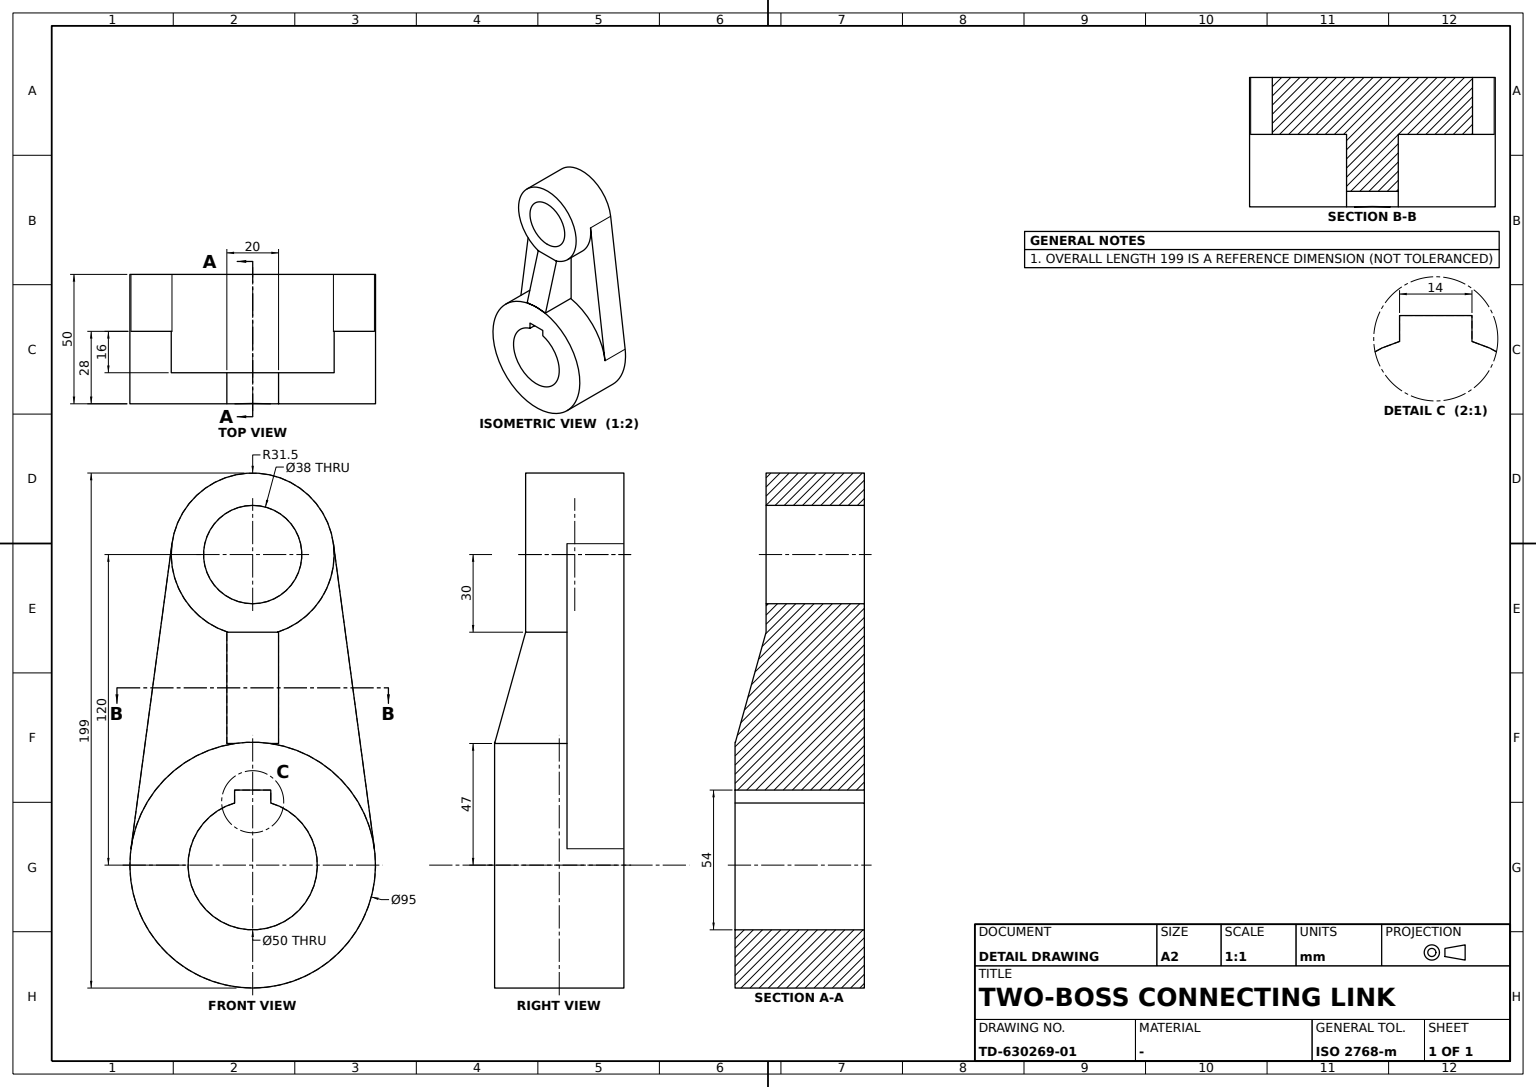
ISO-10303-21;
HEADER;
FILE_DESCRIPTION((''),'2;1');
FILE_NAME('','',(''),(''),'','','');
FILE_SCHEMA(('AUTOMOTIVE_DESIGN'));
ENDSEC;
DATA;
#1=APPLICATION_CONTEXT('');
#2=PRODUCT_CONTEXT('',#1,'mechanical');
#3=PRODUCT('','','',(#2));
#4=PRODUCT_DEFINITION_FORMATION('','',#3);
#5=PRODUCT_DEFINITION_CONTEXT('',#1,'design');
#6=PRODUCT_DEFINITION('','',#4,#5);
#7=PRODUCT_DEFINITION_SHAPE('','',#6);
#8=(LENGTH_UNIT()NAMED_UNIT(*)SI_UNIT(.MILLI.,.METRE.));
#9=(NAMED_UNIT(*)PLANE_ANGLE_UNIT()SI_UNIT($,.RADIAN.));
#10=(NAMED_UNIT(*)SI_UNIT($,.STERADIAN.)SOLID_ANGLE_UNIT());
#11=UNCERTAINTY_MEASURE_WITH_UNIT(LENGTH_MEASURE(0.005),#8,'distance_accuracy_value','');
#12=(GEOMETRIC_REPRESENTATION_CONTEXT(3)GLOBAL_UNCERTAINTY_ASSIGNED_CONTEXT((#11))GLOBAL_UNIT_ASSIGNED_CONTEXT((#8,#9,#10))REPRESENTATION_CONTEXT('',''));
#13=CARTESIAN_POINT('',(-25.,47.075884,6.333333));
#14=VERTEX_POINT('',#13);
#15=CARTESIAN_POINT('',(-3.,47.075884,6.333333));
#16=VERTEX_POINT('',#15);
#17=CARTESIAN_POINT('',(0.,47.075884,6.333333));
#18=DIRECTION('',(1.,0.,0.));
#19=VECTOR('',#18,1000.);
#20=LINE('',#17,#19);
#21=EDGE_CURVE('',#14,#16,#20,.T.);
#22=ORIENTED_EDGE('',*,*,#21,.F.);
#23=CARTESIAN_POINT('',(-25.,31.218744,124.2));
#24=VERTEX_POINT('',#23);
#25=DIRECTION('',(0.,-0.133333333,0.99107125));
#26=VECTOR('',#25,1000.);
#27=LINE('',#13,#26);
#28=EDGE_CURVE('',#14,#24,#27,.T.);
#29=ORIENTED_EDGE('',*,*,#28,.T.);
#30=CARTESIAN_POINT('',(-3.,31.218744,124.2));
#31=VERTEX_POINT('',#30);
#32=CARTESIAN_POINT('',(5.,31.218744,124.2));
#33=LINE('',#32,#19);
#34=EDGE_CURVE('',#24,#31,#33,.T.);
#35=ORIENTED_EDGE('',*,*,#34,.T.);
#36=LINE('',#15,#26);
#37=EDGE_CURVE('',#16,#31,#36,.T.);
#38=ORIENTED_EDGE('',*,*,#37,.F.);
#39=EDGE_LOOP('',(#22,#29,#35,#38));
#40=FACE_BOUND('',#39,.T.);
#41=DIRECTION('',(0.,0.99107125,0.133333333));
#42=AXIS2_PLACEMENT_3D('',#13,#41,#25);
#43=PLANE('',#42);
#44=ADVANCED_FACE('',(#40),#43,.T.);
#45=CARTESIAN_POINT('',(-25.,-31.218744,124.2));
#46=VERTEX_POINT('',#45);
#47=CARTESIAN_POINT('',(-3.,-31.218744,124.2));
#48=VERTEX_POINT('',#47);
#49=CARTESIAN_POINT('',(5.,-31.218744,124.2));
#50=LINE('',#49,#19);
#51=EDGE_CURVE('',#46,#48,#50,.T.);
#52=ORIENTED_EDGE('',*,*,#51,.T.);
#53=CARTESIAN_POINT('',(-3.,-9.604686,90.));
#54=VERTEX_POINT('',#53);
#55=CARTESIAN_POINT('',(-3.,0.,120.));
#56=DIRECTION('',(-1.,0.,0.));
#57=DIRECTION('',(0.,0.,1.));
#58=AXIS2_PLACEMENT_3D('',#55,#56,#57);
#59=CIRCLE('',#58,31.5);
#60=EDGE_CURVE('',#48,#54,#59,.F.);
#61=ORIENTED_EDGE('',*,*,#60,.T.);
#62=CARTESIAN_POINT('',(13.,-9.604686,90.));
#63=VERTEX_POINT('',#62);
#64=LINE('',#53,#19);
#65=EDGE_CURVE('',#63,#54,#64,.F.);
#66=ORIENTED_EDGE('',*,*,#65,.F.);
#67=CARTESIAN_POINT('',(13.,9.604686,90.));
#68=VERTEX_POINT('',#67);
#69=CARTESIAN_POINT('',(13.,0.,120.));
#70=DIRECTION('',(0.,0.,-1.));
#71=AXIS2_PLACEMENT_3D('',#69,#18,#70);
#72=CIRCLE('',#71,31.5);
#73=EDGE_CURVE('',#68,#63,#72,.T.);
#74=ORIENTED_EDGE('',*,*,#73,.F.);
#75=CARTESIAN_POINT('',(-3.,9.604686,90.));
#76=VERTEX_POINT('',#75);
#77=LINE('',#75,#19);
#78=EDGE_CURVE('',#76,#68,#77,.T.);
#79=ORIENTED_EDGE('',*,*,#78,.F.);
#80=EDGE_CURVE('',#76,#31,#59,.F.);
#81=ORIENTED_EDGE('',*,*,#80,.T.);
#82=ORIENTED_EDGE('',*,*,#34,.F.);
#83=CARTESIAN_POINT('',(-25.,0.,120.));
#84=AXIS2_PLACEMENT_3D('',#83,#18,#70);
#85=CIRCLE('',#84,31.5);
#86=EDGE_CURVE('',#46,#24,#85,.F.);
#87=ORIENTED_EDGE('',*,*,#86,.F.);
#88=EDGE_LOOP('',(#52,#61,#66,#74,#79,#81,#82,#87));
#89=FACE_BOUND('',#88,.T.);
#90=CARTESIAN_POINT('',(5.,0.,120.));
#91=DIRECTION('',(0.,1.,0.));
#92=AXIS2_PLACEMENT_3D('',#90,#18,#91);
#93=CYLINDRICAL_SURFACE('',#92,31.5);
#94=ADVANCED_FACE('',(#89),#93,.T.);
#95=CARTESIAN_POINT('',(25.,-10.,47.));
#96=VERTEX_POINT('',#95);
#97=CARTESIAN_POINT('',(-3.,-10.,47.));
#98=VERTEX_POINT('',#97);
#99=CARTESIAN_POINT('',(0.,-10.,47.));
#100=VECTOR('',#56,1000.);
#101=LINE('',#99,#100);
#102=EDGE_CURVE('',#96,#98,#101,.T.);
#103=ORIENTED_EDGE('',*,*,#102,.F.);
#104=CARTESIAN_POINT('',(13.,-10.,90.));
#105=VERTEX_POINT('',#104);
#106=CARTESIAN_POINT('',(35.362268,-10.,9.86854));
#107=DIRECTION('',(0.268798968,0.,-0.963196301));
#108=VECTOR('',#107,1000.);
#109=LINE('',#106,#108);
#110=EDGE_CURVE('',#105,#96,#109,.T.);
#111=ORIENTED_EDGE('',*,*,#110,.F.);
#112=CARTESIAN_POINT('',(-3.,-10.,90.));
#113=VERTEX_POINT('',#112);
#114=CARTESIAN_POINT('',(0.,-10.,90.));
#115=LINE('',#114,#19);
#116=EDGE_CURVE('',#113,#105,#115,.T.);
#117=ORIENTED_EDGE('',*,*,#116,.F.);
#118=CARTESIAN_POINT('',(-3.,-10.,0.));
#119=VECTOR('',#57,1000.);
#120=LINE('',#118,#119);
#121=EDGE_CURVE('',#98,#113,#120,.T.);
#122=ORIENTED_EDGE('',*,*,#121,.F.);
#123=EDGE_LOOP('',(#103,#111,#117,#122));
#124=FACE_BOUND('',#123,.T.);
#125=CARTESIAN_POINT('',(0.,-10.,0.));
#126=AXIS2_PLACEMENT_3D('',#125,#91,#56);
#127=PLANE('',#126);
#128=ADVANCED_FACE('',(#124),#127,.F.);
#129=CARTESIAN_POINT('',(-25.,0.,101.));
#130=VERTEX_POINT('',#129);
#131=CIRCLE('',#84,19.);
#132=EDGE_CURVE('',#130,#130,#131,.T.);
#133=ORIENTED_EDGE('',*,*,#132,.T.);
#134=EDGE_LOOP('',(#133));
#135=FACE_BOUND('',#134,.T.);
#136=CARTESIAN_POINT('',(-25.,7.,29.));
#137=VERTEX_POINT('',#136);
#138=CARTESIAN_POINT('',(-25.,7.,24.));
#139=VERTEX_POINT('',#138);
#140=CARTESIAN_POINT('',(-25.,7.,0.));
#141=VECTOR('',#70,1000.);
#142=LINE('',#140,#141);
#143=EDGE_CURVE('',#137,#139,#142,.T.);
#144=ORIENTED_EDGE('',*,*,#143,.F.);
#145=CARTESIAN_POINT('',(-25.,-7.,29.));
#146=VERTEX_POINT('',#145);
#147=CARTESIAN_POINT('',(-25.,0.,29.));
#148=VECTOR('',#91,1000.);
#149=LINE('',#147,#148);
#150=EDGE_CURVE('',#146,#137,#149,.T.);
#151=ORIENTED_EDGE('',*,*,#150,.F.);
#152=CARTESIAN_POINT('',(-25.,-7.,24.));
#153=VERTEX_POINT('',#152);
#154=CARTESIAN_POINT('',(-25.,-7.,0.));
#155=LINE('',#154,#119);
#156=EDGE_CURVE('',#153,#146,#155,.T.);
#157=ORIENTED_EDGE('',*,*,#156,.F.);
#158=CARTESIAN_POINT('',(-25.,0.,0.));
#159=AXIS2_PLACEMENT_3D('',#158,#18,#70);
#160=CIRCLE('',#159,25.);
#161=EDGE_CURVE('',#153,#139,#160,.T.);
#162=ORIENTED_EDGE('',*,*,#161,.T.);
#163=EDGE_LOOP('',(#144,#151,#157,#162));
#164=FACE_BOUND('',#163,.T.);
#165=ORIENTED_EDGE('',*,*,#28,.F.);
#166=CARTESIAN_POINT('',(-25.,-47.075884,6.333333));
#167=VERTEX_POINT('',#166);
#168=CIRCLE('',#159,47.5);
#169=EDGE_CURVE('',#167,#14,#168,.T.);
#170=ORIENTED_EDGE('',*,*,#169,.F.);
#171=DIRECTION('',(0.,-0.133333333,-0.99107125));
#172=VECTOR('',#171,1000.);
#173=LINE('',#166,#172);
#174=EDGE_CURVE('',#46,#167,#173,.T.);
#175=ORIENTED_EDGE('',*,*,#174,.F.);
#176=ORIENTED_EDGE('',*,*,#86,.T.);
#177=EDGE_LOOP('',(#165,#170,#175,#176));
#178=FACE_BOUND('',#177,.T.);
#179=AXIS2_PLACEMENT_3D('',#158,#18,#91);
#180=PLANE('',#179);
#181=ADVANCED_FACE('',(#135,#164,#178),#180,.F.);
#182=CARTESIAN_POINT('',(13.,10.,90.));
#183=VERTEX_POINT('',#182);
#184=CARTESIAN_POINT('',(13.,0.,90.));
#185=LINE('',#184,#148);
#186=EDGE_CURVE('',#68,#183,#185,.T.);
#187=ORIENTED_EDGE('',*,*,#186,.T.);
#188=CARTESIAN_POINT('',(-3.,10.,90.));
#189=VERTEX_POINT('',#188);
#190=CARTESIAN_POINT('',(0.,10.,90.));
#191=LINE('',#190,#19);
#192=EDGE_CURVE('',#189,#183,#191,.T.);
#193=ORIENTED_EDGE('',*,*,#192,.F.);
#194=CARTESIAN_POINT('',(-3.,0.,90.));
#195=LINE('',#194,#148);
#196=EDGE_CURVE('',#76,#189,#195,.T.);
#197=ORIENTED_EDGE('',*,*,#196,.F.);
#198=ORIENTED_EDGE('',*,*,#78,.T.);
#199=EDGE_LOOP('',(#187,#193,#197,#198));
#200=FACE_BOUND('',#199,.T.);
#201=AXIS2_PLACEMENT_3D('',#194,#57,#18);
#202=PLANE('',#201);
#203=ADVANCED_FACE('',(#200),#202,.T.);
#204=CARTESIAN_POINT('',(-3.,-47.075884,6.333333));
#205=VERTEX_POINT('',#204);
#206=LINE('',#47,#172);
#207=EDGE_CURVE('',#48,#205,#206,.T.);
#208=ORIENTED_EDGE('',*,*,#207,.T.);
#209=CARTESIAN_POINT('',(-3.,-6.873864,47.));
#210=VERTEX_POINT('',#209);
#211=CARTESIAN_POINT('',(-3.,0.,0.));
#212=AXIS2_PLACEMENT_3D('',#211,#56,#57);
#213=CIRCLE('',#212,47.5);
#214=EDGE_CURVE('',#205,#210,#213,.T.);
#215=ORIENTED_EDGE('',*,*,#214,.T.);
#216=CARTESIAN_POINT('',(-3.,0.,47.));
#217=LINE('',#216,#148);
#218=EDGE_CURVE('',#98,#210,#217,.T.);
#219=ORIENTED_EDGE('',*,*,#218,.F.);
#220=ORIENTED_EDGE('',*,*,#121,.T.);
#221=EDGE_CURVE('',#113,#54,#195,.T.);
#222=ORIENTED_EDGE('',*,*,#221,.T.);
#223=ORIENTED_EDGE('',*,*,#60,.F.);
#224=EDGE_LOOP('',(#208,#215,#219,#220,#222,#223));
#225=FACE_BOUND('',#224,.T.);
#226=DIRECTION('',(0.,-1.,0.));
#227=AXIS2_PLACEMENT_3D('',#211,#56,#226);
#228=PLANE('',#227);
#229=ADVANCED_FACE('',(#225),#228,.F.);
#230=EDGE_CURVE('',#63,#68,#185,.T.);
#231=ORIENTED_EDGE('',*,*,#230,.T.);
#232=ORIENTED_EDGE('',*,*,#73,.T.);
#233=EDGE_LOOP('',(#231,#232));
#234=FACE_BOUND('',#233,.T.);
#235=CARTESIAN_POINT('',(13.,0.,101.));
#236=VERTEX_POINT('',#235);
#237=CIRCLE('',#71,19.);
#238=EDGE_CURVE('',#236,#236,#237,.T.);
#239=ORIENTED_EDGE('',*,*,#238,.F.);
#240=EDGE_LOOP('',(#239));
#241=FACE_BOUND('',#240,.T.);
#242=CARTESIAN_POINT('',(13.,0.,0.));
#243=AXIS2_PLACEMENT_3D('',#242,#18,#91);
#244=PLANE('',#243);
#245=ADVANCED_FACE('',(#234,#241),#244,.T.);
#246=ORIENTED_EDGE('',*,*,#230,.F.);
#247=EDGE_CURVE('',#105,#63,#185,.T.);
#248=ORIENTED_EDGE('',*,*,#247,.F.);
#249=ORIENTED_EDGE('',*,*,#110,.T.);
#250=CARTESIAN_POINT('',(25.,-6.873864,47.));
#251=VERTEX_POINT('',#250);
#252=CARTESIAN_POINT('',(25.,0.,47.));
#253=LINE('',#252,#148);
#254=EDGE_CURVE('',#96,#251,#253,.T.);
#255=ORIENTED_EDGE('',*,*,#254,.T.);
#256=CARTESIAN_POINT('',(25.,6.873864,47.));
#257=VERTEX_POINT('',#256);
#258=CARTESIAN_POINT('',(38.116279,0.,0.));
#259=DIRECTION('',(0.963196301,0.,0.268798968));
#260=AXIS2_PLACEMENT_3D('',#258,#259,#107);
#261=ELLIPSE('',#260,49.314973,47.5);
#262=EDGE_CURVE('',#257,#251,#261,.T.);
#263=ORIENTED_EDGE('',*,*,#262,.F.);
#264=CARTESIAN_POINT('',(25.,10.,47.));
#265=VERTEX_POINT('',#264);
#266=EDGE_CURVE('',#257,#265,#253,.T.);
#267=ORIENTED_EDGE('',*,*,#266,.T.);
#268=CARTESIAN_POINT('',(35.362268,10.,9.86854));
#269=LINE('',#268,#108);
#270=EDGE_CURVE('',#183,#265,#269,.T.);
#271=ORIENTED_EDGE('',*,*,#270,.F.);
#272=ORIENTED_EDGE('',*,*,#186,.F.);
#273=EDGE_LOOP('',(#246,#248,#249,#255,#263,#267,#271,#272));
#274=FACE_BOUND('',#273,.T.);
#275=AXIS2_PLACEMENT_3D('',#184,#259,#107);
#276=PLANE('',#275);
#277=ADVANCED_FACE('',(#274),#276,.T.);
#278=CARTESIAN_POINT('',(25.,0.,0.));
#279=AXIS2_PLACEMENT_3D('',#278,#18,#70);
#280=CIRCLE('',#279,47.5);
#281=EDGE_CURVE('',#257,#251,#280,.T.);
#282=ORIENTED_EDGE('',*,*,#281,.F.);
#283=ORIENTED_EDGE('',*,*,#262,.T.);
#284=EDGE_LOOP('',(#282,#283));
#285=FACE_BOUND('',#284,.T.);
#286=CARTESIAN_POINT('',(0.,0.,0.));
#287=AXIS2_PLACEMENT_3D('',#286,#18,#91);
#288=CYLINDRICAL_SURFACE('',#287,47.5);
#289=ADVANCED_FACE('',(#285),#288,.T.);
#290=CARTESIAN_POINT('',(0.,-47.075884,6.333333));
#291=LINE('',#290,#19);
#292=EDGE_CURVE('',#167,#205,#291,.T.);
#293=ORIENTED_EDGE('',*,*,#292,.T.);
#294=ORIENTED_EDGE('',*,*,#207,.F.);
#295=ORIENTED_EDGE('',*,*,#51,.F.);
#296=ORIENTED_EDGE('',*,*,#174,.T.);
#297=EDGE_LOOP('',(#293,#294,#295,#296));
#298=FACE_BOUND('',#297,.T.);
#299=DIRECTION('',(0.,-0.99107125,0.133333333));
#300=AXIS2_PLACEMENT_3D('',#45,#299,#171);
#301=PLANE('',#300);
#302=ADVANCED_FACE('',(#298),#301,.T.);
#303=ORIENTED_EDGE('',*,*,#169,.T.);
#304=ORIENTED_EDGE('',*,*,#21,.T.);
#305=CARTESIAN_POINT('',(-3.,6.873864,47.));
#306=VERTEX_POINT('',#305);
#307=EDGE_CURVE('',#306,#16,#213,.T.);
#308=ORIENTED_EDGE('',*,*,#307,.F.);
#309=LINE('',#256,#19);
#310=EDGE_CURVE('',#306,#257,#309,.T.);
#311=ORIENTED_EDGE('',*,*,#310,.T.);
#312=EDGE_CURVE('',#251,#257,#280,.T.);
#313=ORIENTED_EDGE('',*,*,#312,.F.);
#314=LINE('',#250,#19);
#315=EDGE_CURVE('',#251,#210,#314,.F.);
#316=ORIENTED_EDGE('',*,*,#315,.T.);
#317=ORIENTED_EDGE('',*,*,#214,.F.);
#318=ORIENTED_EDGE('',*,*,#292,.F.);
#319=EDGE_LOOP('',(#303,#304,#308,#311,#313,#316,#317,#318));
#320=FACE_BOUND('',#319,.T.);
#321=ADVANCED_FACE('',(#320),#288,.T.);
#322=CARTESIAN_POINT('',(25.,-7.,24.));
#323=VERTEX_POINT('',#322);
#324=LINE('',#152,#19);
#325=EDGE_CURVE('',#153,#323,#324,.T.);
#326=ORIENTED_EDGE('',*,*,#325,.F.);
#327=ORIENTED_EDGE('',*,*,#156,.T.);
#328=CARTESIAN_POINT('',(25.,-7.,29.));
#329=VERTEX_POINT('',#328);
#330=CARTESIAN_POINT('',(0.,-7.,29.));
#331=LINE('',#330,#19);
#332=EDGE_CURVE('',#146,#329,#331,.T.);
#333=ORIENTED_EDGE('',*,*,#332,.T.);
#334=CARTESIAN_POINT('',(25.,-7.,0.));
#335=LINE('',#334,#119);
#336=EDGE_CURVE('',#323,#329,#335,.T.);
#337=ORIENTED_EDGE('',*,*,#336,.F.);
#338=EDGE_LOOP('',(#326,#327,#333,#337));
#339=FACE_BOUND('',#338,.T.);
#340=CARTESIAN_POINT('',(0.,-7.,24.));
#341=AXIS2_PLACEMENT_3D('',#340,#91,#57);
#342=PLANE('',#341);
#343=ADVANCED_FACE('',(#339),#342,.T.);
#344=CARTESIAN_POINT('',(25.,7.,29.));
#345=VERTEX_POINT('',#344);
#346=CARTESIAN_POINT('',(0.,7.,29.));
#347=LINE('',#346,#19);
#348=EDGE_CURVE('',#137,#345,#347,.T.);
#349=ORIENTED_EDGE('',*,*,#348,.T.);
#350=CARTESIAN_POINT('',(25.,0.,29.));
#351=LINE('',#350,#148);
#352=EDGE_CURVE('',#329,#345,#351,.T.);
#353=ORIENTED_EDGE('',*,*,#352,.F.);
#354=ORIENTED_EDGE('',*,*,#332,.F.);
#355=ORIENTED_EDGE('',*,*,#150,.T.);
#356=EDGE_LOOP('',(#349,#353,#354,#355));
#357=FACE_BOUND('',#356,.T.);
#358=AXIS2_PLACEMENT_3D('',#330,#70,#91);
#359=PLANE('',#358);
#360=ADVANCED_FACE('',(#357),#359,.T.);
#361=ORIENTED_EDGE('',*,*,#238,.T.);
#362=EDGE_LOOP('',(#361));
#363=FACE_BOUND('',#362,.T.);
#364=ORIENTED_EDGE('',*,*,#132,.F.);
#365=EDGE_LOOP('',(#364));
#366=FACE_BOUND('',#365,.T.);
#367=CYLINDRICAL_SURFACE('',#92,19.);
#368=ADVANCED_FACE('',(#363,#366),#367,.F.);
#369=ORIENTED_EDGE('',*,*,#218,.T.);
#370=ORIENTED_EDGE('',*,*,#315,.F.);
#371=ORIENTED_EDGE('',*,*,#254,.F.);
#372=ORIENTED_EDGE('',*,*,#102,.T.);
#373=EDGE_LOOP('',(#369,#370,#371,#372));
#374=FACE_BOUND('',#373,.T.);
#375=AXIS2_PLACEMENT_3D('',#252,#70,#56);
#376=PLANE('',#375);
#377=ADVANCED_FACE('',(#374),#376,.T.);
#378=ORIENTED_EDGE('',*,*,#116,.T.);
#379=ORIENTED_EDGE('',*,*,#247,.T.);
#380=ORIENTED_EDGE('',*,*,#65,.T.);
#381=ORIENTED_EDGE('',*,*,#221,.F.);
#382=EDGE_LOOP('',(#378,#379,#380,#381));
#383=FACE_BOUND('',#382,.T.);
#384=ADVANCED_FACE('',(#383),#202,.T.);
#385=ORIENTED_EDGE('',*,*,#266,.F.);
#386=ORIENTED_EDGE('',*,*,#310,.F.);
#387=CARTESIAN_POINT('',(-3.,10.,47.));
#388=VERTEX_POINT('',#387);
#389=EDGE_CURVE('',#306,#388,#217,.T.);
#390=ORIENTED_EDGE('',*,*,#389,.T.);
#391=CARTESIAN_POINT('',(0.,10.,47.));
#392=LINE('',#391,#100);
#393=EDGE_CURVE('',#265,#388,#392,.T.);
#394=ORIENTED_EDGE('',*,*,#393,.F.);
#395=EDGE_LOOP('',(#385,#386,#390,#394));
#396=FACE_BOUND('',#395,.T.);
#397=ADVANCED_FACE('',(#396),#376,.T.);
#398=ORIENTED_EDGE('',*,*,#312,.T.);
#399=ORIENTED_EDGE('',*,*,#281,.T.);
#400=EDGE_LOOP('',(#398,#399));
#401=FACE_BOUND('',#400,.T.);
#402=ORIENTED_EDGE('',*,*,#336,.T.);
#403=ORIENTED_EDGE('',*,*,#352,.T.);
#404=CARTESIAN_POINT('',(25.,7.,24.));
#405=VERTEX_POINT('',#404);
#406=CARTESIAN_POINT('',(25.,7.,0.));
#407=LINE('',#406,#141);
#408=EDGE_CURVE('',#345,#405,#407,.T.);
#409=ORIENTED_EDGE('',*,*,#408,.T.);
#410=CIRCLE('',#279,25.);
#411=EDGE_CURVE('',#323,#405,#410,.T.);
#412=ORIENTED_EDGE('',*,*,#411,.F.);
#413=EDGE_LOOP('',(#402,#403,#409,#412));
#414=FACE_BOUND('',#413,.T.);
#415=AXIS2_PLACEMENT_3D('',#278,#18,#91);
#416=PLANE('',#415);
#417=ADVANCED_FACE('',(#401,#414),#416,.T.);
#418=LINE('',#138,#19);
#419=EDGE_CURVE('',#139,#405,#418,.T.);
#420=ORIENTED_EDGE('',*,*,#419,.F.);
#421=ORIENTED_EDGE('',*,*,#161,.F.);
#422=ORIENTED_EDGE('',*,*,#325,.T.);
#423=ORIENTED_EDGE('',*,*,#411,.T.);
#424=EDGE_LOOP('',(#420,#421,#422,#423));
#425=FACE_BOUND('',#424,.T.);
#426=CYLINDRICAL_SURFACE('',#287,25.);
#427=ADVANCED_FACE('',(#425),#426,.F.);
#428=CARTESIAN_POINT('',(-3.,10.,0.));
#429=LINE('',#428,#119);
#430=EDGE_CURVE('',#388,#189,#429,.T.);
#431=ORIENTED_EDGE('',*,*,#430,.F.);
#432=ORIENTED_EDGE('',*,*,#389,.F.);
#433=ORIENTED_EDGE('',*,*,#307,.T.);
#434=ORIENTED_EDGE('',*,*,#37,.T.);
#435=ORIENTED_EDGE('',*,*,#80,.F.);
#436=ORIENTED_EDGE('',*,*,#196,.T.);
#437=EDGE_LOOP('',(#431,#432,#433,#434,#435,#436));
#438=FACE_BOUND('',#437,.T.);
#439=ADVANCED_FACE('',(#438),#228,.F.);
#440=ORIENTED_EDGE('',*,*,#348,.F.);
#441=ORIENTED_EDGE('',*,*,#143,.T.);
#442=ORIENTED_EDGE('',*,*,#419,.T.);
#443=ORIENTED_EDGE('',*,*,#408,.F.);
#444=EDGE_LOOP('',(#440,#441,#442,#443));
#445=FACE_BOUND('',#444,.T.);
#446=AXIS2_PLACEMENT_3D('',#346,#226,#70);
#447=PLANE('',#446);
#448=ADVANCED_FACE('',(#445),#447,.T.);
#449=ORIENTED_EDGE('',*,*,#393,.T.);
#450=ORIENTED_EDGE('',*,*,#430,.T.);
#451=ORIENTED_EDGE('',*,*,#192,.T.);
#452=ORIENTED_EDGE('',*,*,#270,.T.);
#453=EDGE_LOOP('',(#449,#450,#451,#452));
#454=FACE_BOUND('',#453,.T.);
#455=CARTESIAN_POINT('',(0.,10.,0.));
#456=AXIS2_PLACEMENT_3D('',#455,#91,#56);
#457=PLANE('',#456);
#458=ADVANCED_FACE('',(#454),#457,.T.);
#459=CLOSED_SHELL('',(#44,#94,#128,#181,#203,#229,#245,#277,#289,#302,#321,#343,#360,#368,#377,#384,#397,#417,#427,#439,#448,#458));
#460=MANIFOLD_SOLID_BREP('',#459);
#461=ADVANCED_BREP_SHAPE_REPRESENTATION('',(#460),#12);
#462=SHAPE_DEFINITION_REPRESENTATION(#7,#461);
ENDSEC;
END-ISO-10303-21;
